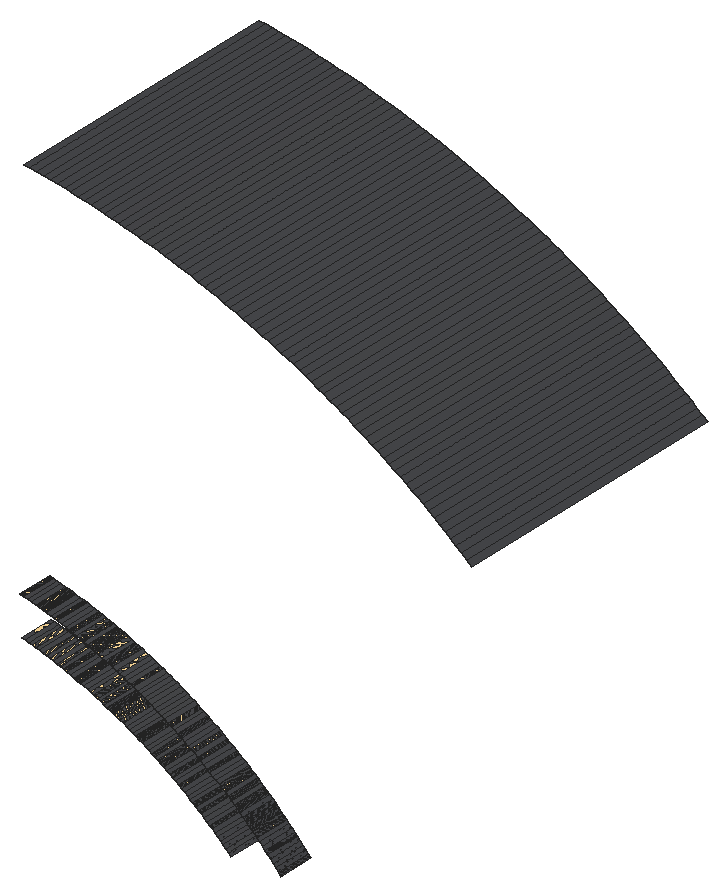
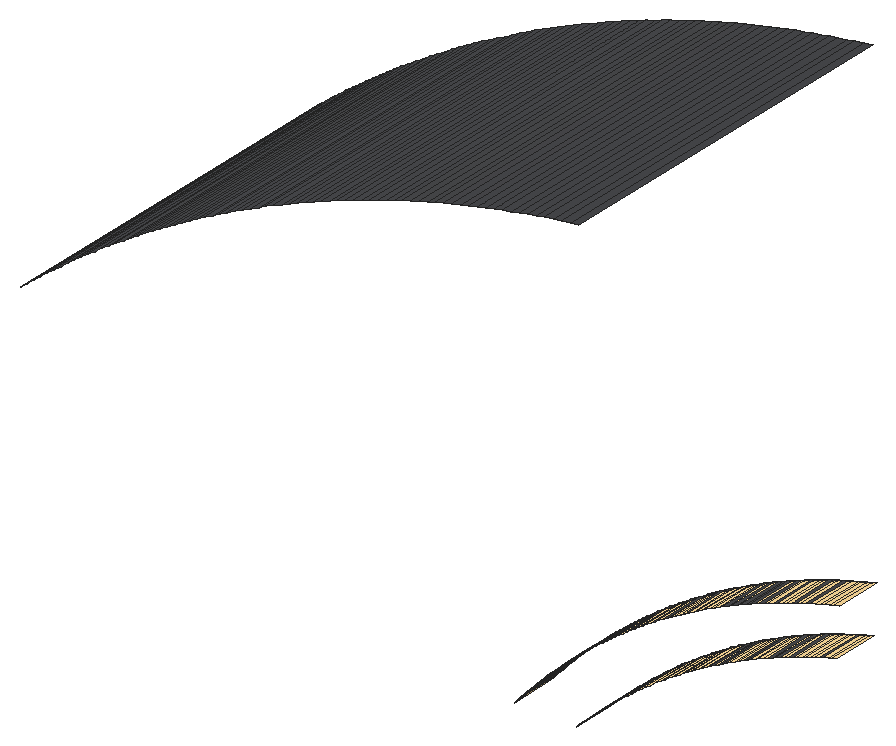
# SketchUp Ruby script. Lengths in inches.
U = 1.inch
M = Sketchup.active_model
def pt(a) = Geom::Point3d.new(a.map { |v| v * U })
def face(e, loops, mat)
  f = e.add_face(loops[0].map { |a| pt(a) })
  loops[1..].each { |l| e.add_face(l.map { |a| pt(a) }).erase! }
  f.material = f.back_material = mat if mat
  f
end
# faces: each face lists its corners as indices into pts; further lists are holes
def faces(e, pts, list, mat = nil) = list.each { |f| face(e, (f[0].is_a?(Array) ? f : [f]).map { |l| l.map { |i| pts[i] } }, mat) }
# xy, xz, yz: faces in a plane at the given z, y or x. An outline is a flat list of corners, or four numbers for a rectangle; further outlines are holes
def ring(l) = l.size == 4 ? [[l[0], l[1]], [l[2], l[1]], [l[2], l[3]], [l[0], l[3]]] : l.each_slice(2).to_a
def flat(e, list, mat, &to3) = list.each { |f| face(e, (f[0].is_a?(Array) ? f : [f]).map { |l| ring(l).map { |u, v| to3.(u, v) } }, mat) }
def xy(e, z, list, mat = nil) = flat(e, list, mat) { |x, y| [x, y, z] }
def xz(e, y, list, mat = nil) = flat(e, list, mat) { |x, z| [x, y, z] }
def yz(e, x, list, mat = nil) = flat(e, list, mat) { |y, z| [x, y, z] }
def lines(e, pts, list) = list.each { |a, b| e.add_line(pt(pts[a]), pt(pts[b])) }
# prism: a flat outline (further loops are holes) pulled along v
def prism(e, loops, v, mat = nil)
  f = face(e, loops, mat); d = Geom::Vector3d.new(v.map { |x| x * U })
  f.pushpull(f.normal.samedirection?(d) ? d.length : -d.length)
end
def box(e, o, s, mat = nil) = prism(e, [[o, [o[0] + s[0], o[1], o[2]], [o[0] + s[0], o[1] + s[1], o[2]], [o[0], o[1] + s[1], o[2]]]], [0, 0, s[2]], mat)
def at(x, y, z, deg = 0) = Geom::Transformation.translation(pt([x, y, z])) * Geom::Transformation.rotation(ORIGIN, Z_AXIS, deg.degrees)
def axes(o, x, y, z) = Geom::Transformation.new([*x, 0, *y, 0, *z, 0, *pt(o).to_a, 1])
def part(name) = M.definitions.add(name)
# library, detail: a bought-in or finely detailed component or shape, given as its bounding box
def library(name, o, s) = part(name).tap { |d| box(d.entities, o, s) }
def detail(e, o, s) = box(e.add_group.entities, o, s)
def put(e, d, t, mat = nil) = e.add_instance(d, t).tap { |i| i.material = mat if mat }
def group(e, t, mat = nil) = e.add_group.tap { |g| g.transformation = t; g.material = mat if mat }.entities
root = M.entities
M.materials.add("1432 AP 8245 TAR ROAD").color = [71, 72, 75]
M.materials.add("Outer Light").color = [251, 217, 152]
p = [[550.44,95.37,574.23],[550.54,95.37,574.12],[550.54,96.87,574.12],[550.44,96.87,574.23],[550.44,96.87,574.23],[550.54,96.87,574.12],
  [550.54,95.37,574.12],[550.44,95.37,574.23],[552.59,95.37,574.11],[552.48,95.37,574.23],[552.48,96.87,574.23],[552.59,96.87,574.11],
  [552.59,96.87,574.11],[552.48,96.87,574.23],[552.48,95.37,574.23],[552.59,95.37,574.11],[550.33,95.37,574.33],[550.33,96.87,574.33],
  [550.33,96.87,574.33],[550.33,95.37,574.33],[552.38,95.37,574.35],[552.38,96.87,574.35],[552.38,96.87,574.35],[552.38,95.37,574.35],
  [550.22,95.37,574.4375],[550.22,96.87,574.4375],[550.22,96.87,574.4375],[550.22,95.37,574.4375],[552.27,95.37,574.47],[552.27,96.87,574.47],
  [552.27,96.87,574.47],[552.27,95.37,574.47],[550.11,95.37,574.54],[550.11,96.87,574.54],[550.11,96.87,574.54],[550.11,95.37,574.54],
  [550.01,95.37,574.64],[550.01,96.87,574.64],[550.01,96.87,574.64],[550.01,95.37,574.64],[552.16,95.37,574.59],[552.16,96.87,574.59],
  [552.16,96.87,574.59],[552.16,95.37,574.59],[549.9,95.37,574.74],[549.9,96.87,574.74],[549.9,96.87,574.74],[549.9,95.37,574.74],
  [552.05,95.37,574.71],[552.05,96.87,574.71],[552.05,96.87,574.71],[552.05,95.37,574.71],[549.79,95.37,574.85],[549.79,96.87,574.85],
  [549.79,96.87,574.85],[549.79,95.37,574.85],[551.94,95.37,574.83],[551.94,96.87,574.83],[551.94,96.87,574.83],[551.94,95.37,574.83],
  [549.68,95.37,574.95],[549.68,96.87,574.95],[549.68,96.87,574.95],[549.68,95.37,574.95],[551.83,95.37,574.94],[551.83,96.87,574.94],
  [551.83,96.87,574.94],[551.83,95.37,574.94],[549.56,95.37,575.04],[549.56,96.87,575.04],[549.56,96.87,575.04],[549.56,95.37,575.04],
  [551.72,95.37,575.06],[551.72,96.87,575.06],[551.72,96.87,575.06],[551.72,95.37,575.06],[549.45,95.37,575.14],[549.45,96.87,575.14],
  [549.45,96.87,575.14],[549.45,95.37,575.14],[549.34,95.37,575.24],[549.34,96.87,575.24],[549.34,96.87,575.24],[549.34,95.37,575.24],
  [551.61,95.37,575.17],[551.61,96.87,575.17],[551.61,96.87,575.17],[551.61,95.37,575.17],[549.23,95.37,575.34],[549.23,96.87,575.34],
  [549.23,96.87,575.34],[549.23,95.37,575.34],[551.5,95.37,575.29],[551.5,96.87,575.29],[551.5,96.87,575.29],[551.5,95.37,575.29],
  [549.11,95.37,575.43],[549.11,96.87,575.43],[549.11,96.87,575.43],[549.11,95.37,575.43],[551.38,95.37,575.4],[551.38,96.87,575.4],
  [551.38,96.87,575.4],[551.38,95.37,575.4],[549,95.37,575.53],[549,96.87,575.53],[549,96.87,575.53],[549,95.37,575.53],
  [551.27,95.37,575.51],[551.27,96.87,575.51],[551.27,96.87,575.51],[551.27,95.37,575.51],[548.88,95.37,575.62],[548.88,96.87,575.62],
  [548.88,96.87,575.62],[548.88,95.37,575.62],[551.15,95.37,575.625],[551.15,96.87,575.625],[551.15,96.87,575.625],[551.15,95.37,575.625],
  [548.76,95.37,575.71],[548.76,96.87,575.71],[548.76,96.87,575.71],[548.76,95.37,575.71],[551.03,95.37,575.74],[551.03,96.87,575.74],
  [551.03,96.87,575.74],[551.03,95.37,575.74],[548.65,95.37,575.8],[548.65,96.87,575.8],[548.65,96.87,575.8],[548.65,95.37,575.8],
  [550.92,95.37,575.85],[550.92,96.87,575.85],[550.92,96.87,575.85],[550.92,95.37,575.85],[548.53,95.37,575.9],[548.53,96.87,575.9],
  [548.53,96.87,575.9],[548.53,95.37,575.9],[550.8,95.37,575.95],[550.8,96.87,575.95],[550.8,96.87,575.95],[550.8,95.37,575.95],
  [548.41,95.37,575.99],[548.41,96.87,575.99],[548.41,96.87,575.99],[548.41,95.37,575.99],[548.29,95.37,576.08],[548.29,96.87,576.08],
  [548.29,96.87,576.08],[548.29,95.37,576.08],[550.68,95.37,576.0625],[550.68,96.87,576.0625],[550.68,96.87,576.0625],[550.68,95.37,576.0625],
  [548.17,95.37,576.16],[548.17,96.87,576.16],[548.17,96.87,576.16],[548.17,95.37,576.16],[550.56,95.37,576.17],[550.56,96.87,576.17],
  [550.56,96.87,576.17],[550.56,95.37,576.17],[548.05,95.37,576.25],[548.05,96.87,576.25],[548.05,96.87,576.25],[548.05,95.37,576.25],
  [550.4375,95.37,576.28],[550.4375,96.87,576.28],[550.4375,96.87,576.28],[550.4375,95.37,576.28],[547.8,95.37,576.42],[547.93,95.37,576.34],
  [547.93,96.87,576.34],[547.8,96.87,576.42],[547.8,96.87,576.42],[547.93,96.87,576.34],[547.93,95.37,576.34],[547.8,95.37,576.42],
  [550.3125,95.37,576.38],[550.3125,96.87,576.38],[550.3125,96.87,576.38],[550.3125,95.37,576.38],[547.68,95.37,576.51],[547.68,96.87,576.51],
  [547.68,96.87,576.51],[547.68,95.37,576.51],[550.19,95.37,576.48],[550.19,96.87,576.48],[550.19,96.87,576.48],[550.19,95.37,576.48],
  [547.56,95.37,576.59],[547.56,96.87,576.59],[547.56,96.87,576.59],[547.56,95.37,576.59],[550.07,95.37,576.59],[550.07,96.87,576.59],
  [550.07,96.87,576.59],[550.07,95.37,576.59],[547.43,95.37,576.67],[547.43,96.87,576.67],[547.43,96.87,576.67],[547.43,95.37,576.67],
  [549.94,95.37,576.69],[549.94,96.87,576.69],[549.94,96.87,576.69],[549.94,95.37,576.69],[547.31,95.37,576.75],[547.31,96.87,576.75],
  [547.31,96.87,576.75],[547.31,95.37,576.75],[549.82,95.37,576.79],[549.82,96.87,576.79],[549.82,96.87,576.79],[549.82,95.37,576.79],
  [547.05,95.37,576.91],[547.18,95.37,576.83],[547.18,96.87,576.83],[547.05,96.87,576.91],[547.05,96.87,576.91],[547.18,96.87,576.83],
  [547.18,95.37,576.83],[547.05,95.37,576.91],[549.69,95.37,576.89],[549.69,96.87,576.89],[549.69,96.87,576.89],[549.69,95.37,576.89],
  [546.93,95.37,576.99],[546.93,96.87,576.99],[546.93,96.87,576.99],[546.93,95.37,576.99],[549.56,95.37,576.99],[549.56,96.87,576.99],
  [549.56,96.87,576.99],[549.56,95.37,576.99],[546.8,95.37,577.07],[546.8,96.87,577.07],[546.8,96.87,577.07],[546.8,95.37,577.07],
  [549.4375,95.37,577.09],[549.4375,96.87,577.09],[549.4375,96.87,577.09],[549.4375,95.37,577.09],[546.54,95.37,577.22],[546.67,95.37,577.15],
  [546.67,96.87,577.15],[546.54,96.87,577.22],[546.54,96.87,577.22],[546.67,96.87,577.15],[546.67,95.37,577.15],[546.54,95.37,577.22],
  [549.31,95.37,577.1875],[549.31,96.87,577.1875],[549.31,96.87,577.1875],[549.31,95.37,577.1875],[546.41,95.37,577.3],[546.41,96.87,577.3],
  [546.41,96.87,577.3],[546.41,95.37,577.3],[549.18,95.37,577.28],[549.18,96.87,577.28],[549.18,96.87,577.28],[549.18,95.37,577.28],
  [546.28,95.37,577.37],[546.28,96.87,577.37],[546.28,96.87,577.37],[546.28,95.37,577.37],[549.05,95.37,577.375],[549.05,96.87,577.375],
  [549.05,96.87,577.375],[549.05,95.37,577.375],[546.02,95.37,577.51],[546.15,95.37,577.44],[546.15,96.87,577.44],[546.02,96.87,577.51],
  [546.02,96.87,577.51],[546.15,96.87,577.44],[546.15,95.37,577.44],[546.02,95.37,577.51],[548.92,95.37,577.47],[548.92,96.87,577.47],
  [548.92,96.87,577.47],[548.92,95.37,577.47],[545.89,95.37,577.58],[545.89,96.87,577.58],[545.89,96.87,577.58],[545.89,95.37,577.58],
  [548.79,95.37,577.5625],[548.79,96.87,577.5625],[548.79,96.87,577.5625],[548.79,95.37,577.5625],[545.76,95.37,577.65],[545.76,96.87,577.65],
  [545.76,96.87,577.65],[545.76,95.37,577.65],[548.66,95.37,577.66],[548.66,96.87,577.66],[548.66,96.87,577.66],[548.66,95.37,577.66],
  [545.49,95.37,577.79],[545.625,95.37,577.72],[545.625,96.87,577.72],[545.49,96.87,577.79],[545.49,96.87,577.79],[545.625,96.87,577.72],
  [545.625,95.37,577.72],[545.49,95.37,577.79],[548.52,95.37,577.75],[548.39,95.37,577.84],[548.39,96.87,577.84],[548.52,96.87,577.75],
  [548.52,96.87,577.75],[548.39,96.87,577.84],[548.39,95.37,577.84],[548.52,95.37,577.75],[545.36,95.37,577.85],[545.36,96.87,577.85],
  [545.36,96.87,577.85],[545.36,95.37,577.85],[548.25,95.37,577.93],[548.25,96.87,577.93],[548.25,96.87,577.93],[548.25,95.37,577.93],
  [545.09,95.37,577.98],[545.22,95.37,577.92],[545.22,96.87,577.92],[545.09,96.87,577.98],[545.09,96.87,577.98],[545.22,96.87,577.92],
  [545.22,95.37,577.92],[545.09,95.37,577.98],[548.12,95.37,578.01],[548.12,96.87,578.01],[548.12,96.87,578.01],[548.12,95.37,578.01],
  [544.82,95.37,578.11],[544.95,95.37,578.05],[544.95,96.87,578.05],[544.82,96.87,578.11],[544.82,96.87,578.11],[544.95,96.87,578.05],
  [544.95,95.37,578.05],[544.82,95.37,578.11],[547.98,95.37,578.1],[547.98,96.87,578.1],[547.98,96.87,578.1],[547.98,95.37,578.1],
  [544.68,95.37,578.17],[544.68,96.87,578.17],[544.68,96.87,578.17],[544.68,95.37,578.17],[547.85,95.37,578.1875],[547.85,96.87,578.1875],
  [547.85,96.87,578.1875],[547.85,95.37,578.1875],[544.41,95.37,578.29],[544.55,95.37,578.23],[544.55,96.87,578.23],[544.41,96.87,578.29],
  [544.41,96.87,578.29],[544.55,96.87,578.23],[544.55,95.37,578.23],[544.41,95.37,578.29],[547.71,95.37,578.27],[547.71,96.87,578.27],
  [547.71,96.87,578.27],[547.71,95.37,578.27],[544.13,95.37,578.4],[544.27,95.37,578.35],[544.27,96.87,578.35],[544.13,96.87,578.4],
  [544.13,96.87,578.4],[544.27,96.87,578.35],[544.27,95.37,578.35],[544.13,95.37,578.4],[547.57,95.37,578.35],[547.57,96.87,578.35],
  [547.57,96.87,578.35],[547.57,95.37,578.35],[543.99,95.37,578.46],[543.99,96.87,578.46],[543.99,96.87,578.46],[543.99,95.37,578.46],
  [547.44,95.37,578.4375],[547.3,95.37,578.52],[547.3,96.87,578.52],[547.44,96.87,578.4375],[547.44,96.87,578.4375],[547.3,96.87,578.52],
  [547.3,95.37,578.52],[547.44,95.37,578.4375],[543.72,95.37,578.57],[543.86,95.37,578.51],[543.86,96.87,578.51],[543.72,96.87,578.57],
  [543.72,96.87,578.57],[543.86,96.87,578.51],[543.86,95.37,578.51],[543.72,95.37,578.57],[547.16,95.37,578.6],[547.16,96.87,578.6],
  [547.16,96.87,578.6],[547.16,95.37,578.6],[543.4375,95.37,578.67],[543.58,95.37,578.62],[543.58,96.87,578.62],[543.4375,96.87,578.67],
  [543.4375,96.87,578.67],[543.58,96.87,578.62],[543.58,95.37,578.62],[543.4375,95.37,578.67],[547.02,95.37,578.68],[547.02,96.87,578.68],
  [547.02,96.87,578.68],[547.02,95.37,578.68],[543.15,95.37,578.77],[543.3,95.37,578.72],[543.3,96.87,578.72],[543.15,96.87,578.77],
  [543.15,96.87,578.77],[543.3,96.87,578.72],[543.3,95.37,578.72],[543.15,95.37,578.77],[546.875,95.37,578.76],[546.875,96.87,578.76],
  [546.875,96.87,578.76],[546.875,95.37,578.76],[542.87,95.37,578.86],[543.01,95.37,578.82],[543.01,96.87,578.82],[542.87,96.87,578.86],
  [542.87,96.87,578.86],[543.01,96.87,578.82],[543.01,95.37,578.82],[542.87,95.37,578.86],[546.73,95.37,578.83],[546.59,95.37,578.91],
  [546.59,96.87,578.91],[546.73,96.87,578.83],[546.73,96.87,578.83],[546.59,96.87,578.91],[546.59,95.37,578.91],[546.73,95.37,578.83],
  [542.59,95.37,578.95],[542.73,95.37,578.91],[542.73,96.87,578.91],[542.59,96.87,578.95],[542.59,96.87,578.95],[542.73,96.87,578.91],
  [542.73,95.37,578.91],[542.59,95.37,578.95],[546.45,95.37,578.98],[546.45,96.87,578.98],[546.45,96.87,578.98],[546.45,95.37,578.98],
  [542.16,95.37,579.08],[542.3,95.37,579.04],[542.3,96.87,579.04],[542.16,96.87,579.08],[542.16,96.87,579.08],[542.3,96.87,579.04],
  [542.3,95.37,579.04],[542.16,95.37,579.08],[542.44,95.37,579],[542.44,96.87,579],[542.44,96.87,579],[542.44,95.37,579],
  [546.31,95.37,579.06],[546.31,96.87,579.06],[546.31,96.87,579.06],[546.31,95.37,579.06],[542.01,95.37,579.12],[542.01,96.87,579.12],
  [542.01,96.87,579.12],[542.01,95.37,579.12],[546.16,95.37,579.13],[546.02,95.37,579.2],[546.02,96.87,579.2],[546.16,96.87,579.13],
  [546.16,96.87,579.13],[546.02,96.87,579.2],[546.02,95.37,579.2],[546.16,95.37,579.13],[545.875,95.37,579.27],[545.875,96.87,579.27],
  [545.875,96.87,579.27],[545.875,95.37,579.27],[545.73,95.37,579.34],[545.58,95.37,579.41],[545.58,96.87,579.41],[545.73,96.87,579.34],
  [545.73,96.87,579.34],[545.58,96.87,579.41],[545.58,95.37,579.41],[545.73,95.37,579.34],[545.4375,95.37,579.48],[545.4375,96.87,579.48],
  [545.4375,96.87,579.48],[545.4375,95.37,579.48],[545.29,95.37,579.54],[545.14,95.37,579.61],[545.14,96.87,579.61],[545.29,96.87,579.54],
  [545.29,96.87,579.54],[545.14,96.87,579.61],[545.14,95.37,579.61],[545.29,95.37,579.54],[544.99,95.37,579.67],[544.99,96.87,579.67],
  [544.99,96.87,579.67],[544.99,95.37,579.67],[544.85,95.37,579.73],[544.7,95.37,579.79],[544.7,96.87,579.79],[544.85,96.87,579.73],
  [544.85,96.87,579.73],[544.7,96.87,579.79],[544.7,95.37,579.79],[544.85,95.37,579.73],[544.55,95.37,579.85],[544.55,96.87,579.85],
  [544.55,96.87,579.85],[544.55,95.37,579.85],[544.4,95.37,579.91],[544.25,95.37,579.97],[544.25,96.87,579.97],[544.4,96.87,579.91],
  [544.4,96.87,579.91],[544.25,96.87,579.97],[544.25,95.37,579.97],[544.4,95.37,579.91],[544.1,95.37,580.02],[543.94,95.37,580.08],
  [543.94,96.87,580.08],[544.1,96.87,580.02],[544.1,96.87,580.02],[543.94,96.87,580.08],[543.94,95.37,580.08],[544.1,95.37,580.02],
  [543.79,95.37,580.13],[543.64,95.37,580.1875],[543.64,96.87,580.1875],[543.79,96.87,580.13],[543.79,96.87,580.13],[543.64,96.87,580.1875],
  [543.64,95.37,580.1875],[543.79,95.37,580.13],[543.49,95.37,580.24],[543.33,95.37,580.29],[543.33,96.87,580.29],[543.49,96.87,580.24],
  [543.49,96.87,580.24],[543.33,96.87,580.29],[543.33,95.37,580.29],[543.49,95.37,580.24],[543.18,95.37,580.34],[543.03,95.37,580.39],
  [543.03,96.87,580.39],[543.18,96.87,580.34],[543.18,96.87,580.34],[543.03,96.87,580.39],[543.03,95.37,580.39],[543.18,95.37,580.34],
  [542.875,95.37,580.43],[542.72,95.37,580.48],[542.72,96.87,580.48],[542.875,96.87,580.43],[542.875,96.87,580.43],[542.72,96.87,580.48],
  [542.72,95.37,580.48],[542.875,95.37,580.43],[542.56,95.37,580.52],[542.41,95.37,580.57],[542.41,96.87,580.57],[542.56,96.87,580.52],
  [542.56,96.87,580.52],[542.41,96.87,580.57],[542.41,95.37,580.57],[542.56,95.37,580.52],[542.1,95.37,580.65],[541.94,95.37,580.6875],
  [541.94,96.87,580.6875],[542.1,96.87,580.65],[542.1,96.87,580.65],[541.94,96.87,580.6875],[541.94,95.37,580.6875],[542.1,95.37,580.65],
  [542.25,95.37,580.61],[542.25,96.87,580.61],[542.25,96.87,580.61],[542.25,95.37,580.61],[560.38,107.37,588.17],[560.16,107.37,588.35],
  [560.16,95.37,588.35],[560.38,95.37,588.17],[559.95,107.37,588.53],[559.95,95.37,588.53],[559.73,107.37,588.71],[559.73,95.37,588.71],
  [559.51,107.37,588.89],[559.51,95.37,588.89],[559.29,107.37,589.0625],[559.29,95.37,589.0625],[559.06,107.37,589.24],[559.06,95.37,589.24],
  [558.84,107.37,589.41],[558.84,95.37,589.41],[558.62,107.37,589.58],[558.62,95.37,589.58],[558.39,107.37,589.75],[558.39,95.37,589.75],
  [558.16,107.37,589.92],[558.16,95.37,589.92],[557.93,107.37,590.08],[557.93,95.37,590.08],[557.7,107.37,590.25],[557.7,95.37,590.25],
  [557.47,107.37,590.41],[557.47,95.37,590.41],[557.24,107.37,590.57],[557.24,95.37,590.57],[557,107.37,590.72],[557,95.37,590.72],
  [556.76,107.37,590.88],[556.76,95.37,590.88],[556.53,107.37,591.04],[556.53,95.37,591.04],[556.29,107.37,591.1875],[556.29,95.37,591.1875],
  [556.05,107.37,591.34],[556.05,95.37,591.34],[555.81,107.37,591.49],[555.81,95.37,591.49],[555.57,107.37,591.63],[555.57,95.37,591.63],
  [555.33,107.37,591.78],[555.33,95.37,591.78],[555.08,107.37,591.92],[555.08,95.37,591.92],[554.84,107.37,592.0625],[554.84,95.37,592.0625],
  [554.59,107.37,592.2],[554.59,95.37,592.2],[554.34,107.37,592.34],[554.34,95.37,592.34],[554.09,107.37,592.47],[554.09,95.37,592.47],
  [553.85,107.37,592.61],[553.85,95.37,592.61],[553.6,107.37,592.74],[553.6,95.37,592.74],[553.34,107.37,592.87],[553.34,95.37,592.87],
  [553.09,107.37,593],[553.09,95.37,593],[552.84,107.37,593.12],[552.84,95.37,593.12],[552.58,107.37,593.24],[552.58,95.37,593.24],
  [552.33,107.37,593.37],[552.33,95.37,593.37],[552.07,107.37,593.49],[552.07,95.37,593.49],[551.81,107.37,593.6],[551.81,95.37,593.6],
  [551.56,107.37,593.72],[551.56,95.37,593.72],[551.3,107.37,593.83],[551.3,95.37,593.83],[551.04,107.37,593.94],[551.04,95.37,593.94],
  [550.78,107.37,594.05],[550.78,95.37,594.05],[550.51,107.37,594.16],[550.51,95.37,594.16],[550.25,107.37,594.26],[550.25,95.37,594.26],
  [549.99,107.37,594.37],[549.99,95.37,594.37],[549.73,107.37,594.47],[549.73,95.37,594.47],[549.46,107.37,594.57],[549.46,95.37,594.57],
  [549.19,107.37,594.66],[549.19,95.37,594.66],[548.93,107.37,594.76],[548.93,95.37,594.76],[548.66,107.37,594.85],[548.66,95.37,594.85],
  [548.39,107.37,594.94],[548.125,107.37,595.03],[548.125,95.37,595.03],[548.39,95.37,594.94],[547.86,107.37,595.12],[547.86,95.37,595.12],
  [547.59,107.37,595.2],[547.59,95.37,595.2],[547.31,107.37,595.28],[547.31,95.37,595.28],[547.04,107.37,595.36],[547.04,95.37,595.36],
  [546.77,107.37,595.44],[546.5,107.37,595.52],[546.5,95.37,595.52],[546.77,95.37,595.44],[546.23,107.37,595.59],[546.23,95.37,595.59],
  [545.95,107.37,595.66],[545.95,95.37,595.66],[545.68,107.37,595.73],[545.4,107.37,595.8],[545.4,95.37,595.8],[545.68,95.37,595.73],
  [545.13,107.37,595.86],[545.13,95.37,595.86],[544.85,107.37,595.93],[544.58,107.37,595.99],[544.58,95.37,595.99],[544.85,95.37,595.93],
  [544.3,107.37,596.04],[544.02,107.37,596.1],[544.02,95.37,596.1],[544.3,95.37,596.04],[543.75,107.37,596.15],[543.75,95.37,596.15],
  [543.47,107.37,596.21],[543.1875,107.37,596.26],[543.1875,95.37,596.26],[543.47,95.37,596.21],[542.63,107.37,596.35],[542.35,107.37,596.39],
  [542.35,95.37,596.39],[542.63,95.37,596.35],[542.91,107.37,596.3],[542.91,95.37,596.3],[542.07,107.37,596.43],[542.07,95.37,596.43]]
faces(root,p,[[0,1,2,3],[8,9,10,11],[16,0,3,17],[9,20,21,10],[24,16,17,25],[20,28,29,21],[32,24,25,33],[36,32,33,37],
  [28,40,41,29],[44,36,37,45],[40,48,49,41],[52,44,45,53],[48,56,57,49],[60,52,53,61],[56,64,65,57],[68,60,61,69],
  [64,72,73,65],[76,68,69,77],[80,76,77,81],[72,84,85,73],[88,80,81,89],[84,92,93,85],[96,88,89,97],[92,100,101,93],
  [104,96,97,105],[100,108,109,101],[112,104,105,113],[108,116,117,109],[120,112,113,121],[116,124,125,117],[128,120,121,129],[124,132,133,125],
  [136,128,129,137],[132,140,141,133],[144,136,137,145],[148,144,145,149],[140,152,153,141],[156,148,149,157],[152,160,161,153],[164,156,157,165],
  [160,168,169,161],[172,173,174,175],[173,164,165,174],[168,180,181,169],[184,172,175,185],[180,188,189,181],[192,184,185,193],[188,196,197,189],
  [200,192,193,201],[196,204,205,197],[208,200,201,209],[204,212,213,205],[216,217,218,219],[217,208,209,218],[212,224,225,213],[228,216,219,229],
  [224,232,233,225],[236,228,229,237],[232,240,241,233],[244,245,246,247],[245,236,237,246],[240,252,253,241],[256,244,247,257],[252,260,261,253],
  [264,256,257,265],[260,268,269,261],[272,273,274,275],[273,264,265,274],[268,280,281,269],[284,272,275,285],[280,288,289,281],[292,284,285,293],
  [288,296,297,289],[300,301,302,303],[301,292,293,302],[308,309,310,311],[296,308,311,297],[316,300,303,317],[309,320,321,310],[324,325,326,327],
  [325,316,317,326],[320,332,333,321],[336,337,338,339],[337,324,327,338],[332,344,345,333],[348,336,339,349],[344,352,353,345],[356,357,358,359],
  [357,348,349,358],[352,364,365,353],[368,369,370,371],[369,356,359,370],[364,376,377,365],[380,368,371,381],[384,385,386,387],[376,384,387,377],
  [392,393,394,395],[393,380,381,394],[385,400,401,386],[404,405,406,407],[405,392,395,406],[400,412,413,401],[416,417,418,419],[417,404,407,418],
  [412,424,425,413],[428,429,430,431],[429,416,419,430],[436,437,438,439],[424,436,439,425],[444,445,446,447],[445,428,431,446],[437,452,453,438],
  [456,457,458,459],[457,464,465,458],[464,444,447,465],[452,468,469,453],[472,456,459,473],[476,477,478,479],[468,476,479,469],[477,484,485,478],
  [488,489,490,491],[484,488,491,485],[489,496,497,490],[500,501,502,503],[496,500,503,497],[501,508,509,502],[512,513,514,515],[508,512,515,509],
  [513,520,521,514],[524,525,526,527],[520,524,527,521],[532,533,534,535],[525,532,535,526],[540,541,542,543],[533,540,543,534],[548,549,550,551],
  [541,548,551,542],[556,557,558,559],[549,556,559,550],[564,565,566,567],[557,564,567,558],[572,573,574,575],[565,572,575,566],[580,581,582,583],
  [588,580,583,589],[573,588,589,574],[592,593,594,595],[593,596,597,594],[596,598,599,597],[598,600,601,599],[600,602,603,601],[602,604,605,603],
  [604,606,607,605],[606,608,609,607],[608,610,611,609],[610,612,613,611],[612,614,615,613],[614,616,617,615],[616,618,619,617],[618,620,621,619],
  [620,622,623,621],[622,624,625,623],[624,626,627,625],[626,628,629,627],[628,630,631,629],[630,632,633,631],[632,634,635,633],[634,636,637,635],
  [636,638,639,637],[638,640,641,639],[640,642,643,641],[642,644,645,643],[644,646,647,645],[646,648,649,647],[648,650,651,649],[650,652,653,651],
  [652,654,655,653],[654,656,657,655],[656,658,659,657],[658,660,661,659],[660,662,663,661],[662,664,665,663],[664,666,667,665],[666,668,669,667],
  [668,670,671,669],[670,672,673,671],[672,674,675,673],[674,676,677,675],[676,678,679,677],[678,680,681,679],[680,682,683,681],[682,684,685,683],
  [684,686,687,685],[686,688,689,687],[690,691,692,693],[688,690,693,689],[691,694,695,692],[694,696,697,695],[696,698,699,697],[698,700,701,699],
  [702,703,704,705],[700,702,705,701],[703,706,707,704],[706,708,709,707],[710,711,712,713],[708,710,713,709],[711,714,715,712],[716,717,718,719],
  [714,716,719,715],[720,721,722,723],[717,720,723,718],[721,724,725,722],[726,727,728,729],[724,726,729,725],[730,731,732,733],[734,730,733,735],
  [727,734,735,728],[731,736,737,732]],"1432 AP 8245 TAR ROAD")
faces(root,p,[[4,5,6,7],[12,13,14,15],[18,4,7,19],[13,22,23,14],[26,18,19,27],[22,30,31,23],[34,26,27,35],[38,34,35,39],
  [30,42,43,31],[46,38,39,47],[42,50,51,43],[54,46,47,55],[50,58,59,51],[62,54,55,63],[58,66,67,59],[70,62,63,71],
  [66,74,75,67],[78,70,71,79],[82,78,79,83],[74,86,87,75],[90,82,83,91],[86,94,95,87],[98,90,91,99],[94,102,103,95],
  [106,98,99,107],[102,110,111,103],[114,106,107,115],[110,118,119,111],[122,114,115,123],[118,126,127,119],[130,122,123,131],[126,134,135,127],
  [138,130,131,139],[134,142,143,135],[146,138,139,147],[150,146,147,151],[142,154,155,143],[158,150,151,159],[154,162,163,155],[166,158,159,167],
  [162,170,171,163],[176,177,178,179],[177,166,167,178],[170,182,183,171],[186,176,179,187],[182,190,191,183],[194,186,187,195],[190,198,199,191],
  [202,194,195,203],[198,206,207,199],[210,202,203,211],[206,214,215,207],[220,221,222,223],[221,210,211,222],[214,226,227,215],[230,220,223,231],
  [226,234,235,227],[238,230,231,239],[234,242,243,235],[248,249,250,251],[249,238,239,250],[242,254,255,243],[258,248,251,259],[254,262,263,255],
  [266,258,259,267],[262,270,271,263],[276,277,278,279],[277,266,267,278],[270,282,283,271],[286,276,279,287],[282,290,291,283],[294,286,287,295],
  [290,298,299,291],[304,305,306,307],[305,294,295,306],[312,313,314,315],[298,312,315,299],[318,304,307,319],[313,322,323,314],[328,329,330,331],
  [329,318,319,330],[322,334,335,323],[340,341,342,343],[341,328,331,342],[334,346,347,335],[350,340,343,351],[346,354,355,347],[360,361,362,363],
  [361,350,351,362],[354,366,367,355],[372,373,374,375],[373,360,363,374],[366,378,379,367],[382,372,375,383],[388,389,390,391],[378,388,391,379],
  [396,397,398,399],[397,382,383,398],[389,402,403,390],[408,409,410,411],[409,396,399,410],[402,414,415,403],[420,421,422,423],[421,408,411,422],
  [414,426,427,415],[432,433,434,435],[433,420,423,434],[440,441,442,443],[426,440,443,427],[448,449,450,451],[449,432,435,450],[441,454,455,442],
  [460,461,462,463],[461,466,467,462],[466,448,451,467],[454,470,471,455],[474,460,463,475],[480,481,482,483],[470,480,483,471],[481,486,487,482],
  [492,493,494,495],[486,492,495,487],[493,498,499,494],[504,505,506,507],[498,504,507,499],[505,510,511,506],[516,517,518,519],[510,516,519,511],
  [517,522,523,518],[528,529,530,531],[522,528,531,523],[536,537,538,539],[529,536,539,530],[544,545,546,547],[537,544,547,538],[552,553,554,555],
  [545,552,555,546],[560,561,562,563],[553,560,563,554],[568,569,570,571],[561,568,571,562],[576,577,578,579],[569,576,579,570],[584,585,586,587],
  [590,584,587,591],[577,590,591,578]],"Outer Light")
